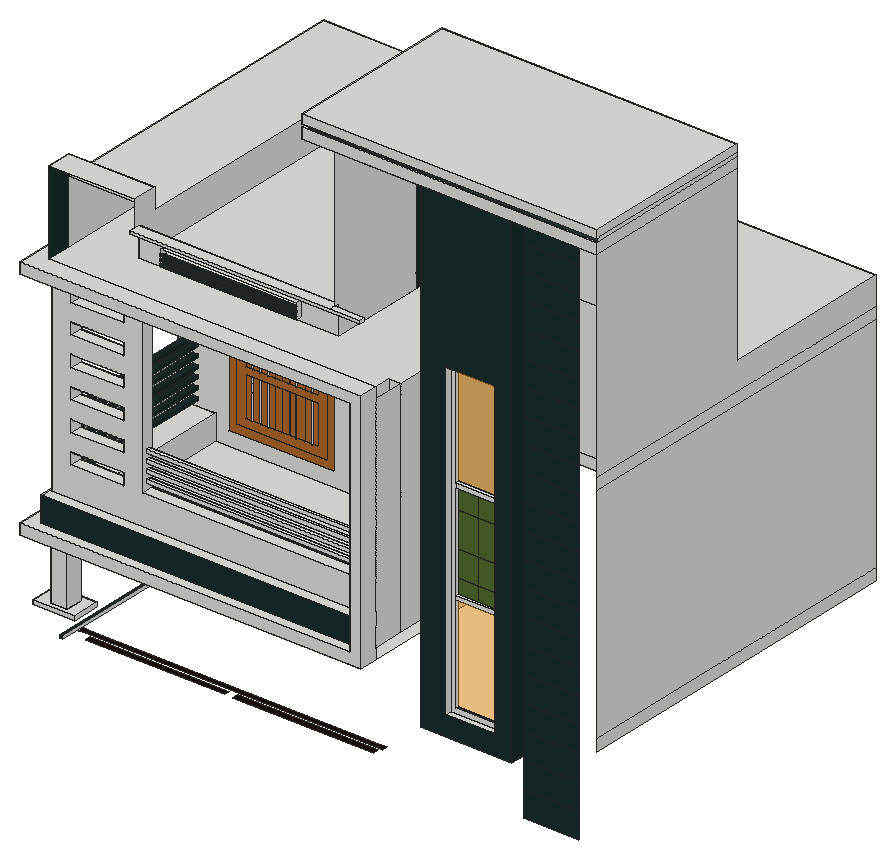
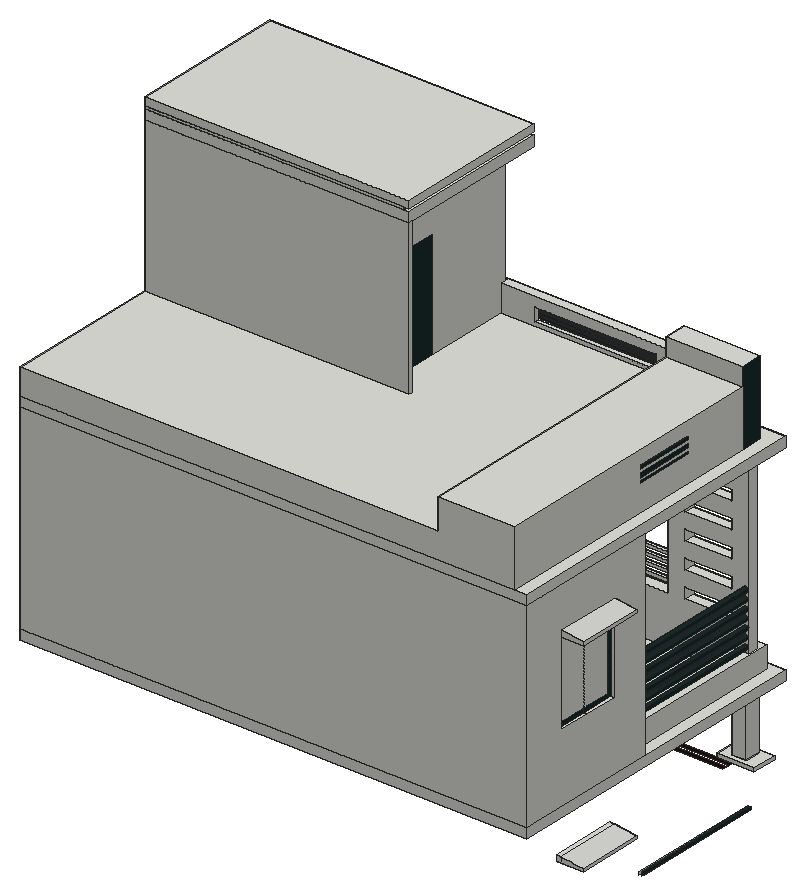
# SketchUp Ruby script. Lengths in inches.
U = 1.inch
M = Sketchup.active_model
def pt(a) = Geom::Point3d.new(a.map { |v| v * U })
def face(e, loops, mat)
  f = e.add_face(loops[0].map { |a| pt(a) })
  loops[1..].each { |l| e.add_face(l.map { |a| pt(a) }).erase! }
  f.material = f.back_material = mat if mat
  f
end
# faces: each face lists its corners as indices into pts; further lists are holes
def faces(e, pts, list, mat = nil) = list.each { |f| face(e, (f[0].is_a?(Array) ? f : [f]).map { |l| l.map { |i| pts[i] } }, mat) }
# xy, xz, yz: faces in a plane at the given z, y or x. An outline is a flat list of corners, or four numbers for a rectangle; further outlines are holes
def ring(l) = l.size == 4 ? [[l[0], l[1]], [l[2], l[1]], [l[2], l[3]], [l[0], l[3]]] : l.each_slice(2).to_a
def flat(e, list, mat, &to3) = list.each { |f| face(e, (f[0].is_a?(Array) ? f : [f]).map { |l| ring(l).map { |u, v| to3.(u, v) } }, mat) }
def xy(e, z, list, mat = nil) = flat(e, list, mat) { |x, y| [x, y, z] }
def xz(e, y, list, mat = nil) = flat(e, list, mat) { |x, z| [x, y, z] }
def yz(e, x, list, mat = nil) = flat(e, list, mat) { |y, z| [x, y, z] }
def lines(e, pts, list) = list.each { |a, b| e.add_line(pt(pts[a]), pt(pts[b])) }
# prism: a flat outline (further loops are holes) pulled along v
def prism(e, loops, v, mat = nil)
  f = face(e, loops, mat); d = Geom::Vector3d.new(v.map { |x| x * U })
  f.pushpull(f.normal.samedirection?(d) ? d.length : -d.length)
end
def box(e, o, s, mat = nil) = prism(e, [[o, [o[0] + s[0], o[1], o[2]], [o[0] + s[0], o[1] + s[1], o[2]], [o[0], o[1] + s[1], o[2]]]], [0, 0, s[2]], mat)
def at(x, y, z, deg = 0) = Geom::Transformation.translation(pt([x, y, z])) * Geom::Transformation.rotation(ORIGIN, Z_AXIS, deg.degrees)
def axes(o, x, y, z) = Geom::Transformation.new([*x, 0, *y, 0, *z, 0, *pt(o).to_a, 1])
def part(name) = M.definitions.add(name)
# library, detail: a bought-in or finely detailed component or shape, given as its bounding box
def library(name, o, s) = part(name).tap { |d| box(d.entities, o, s) }
def detail(e, o, s) = box(e.add_group.entities, o, s)
def put(e, d, t, mat = nil) = e.add_instance(d, t).tap { |i| i.material = mat if mat }
def group(e, t, mat = nil) = e.add_group.tap { |g| g.transformation = t; g.material = mat if mat }.entities
root = M.entities
M.materials.add("[0056_Yellow]").color = [255, 255, 0]
M.materials.add("[0059_DarkOliveGreen]").color = [85, 107, 47]
M.materials.add("[0078_DarkSlateGray]").color = [27, 45, 45]
M.materials.add("[0078_DarkSlateGray]1").color = [47, 79, 79]
M.materials.add("[Translucent Glass Gray]").color = [255, 153, 0]
M.materials["[Translucent Glass Gray]"].alpha = 0.5
M.materials.add("[Wood Bamboo]").color = [177, 105, 43]
M.materials.add("[Wood Veneer 01]").color = [28, 16, 8]
xy(root,66.44,[[15.47,103.41,17.09,183.375]])
xy(root,68.06,[[15.47,103.41,17.09,185.5625]],"[0078_DarkSlateGray]")
xy(root,77.61,[[37.47,93.625,112.35,96.69],[116.92,93.625,192.625,96.69]],"[Wood Veneer 01]")
xy(root,80.73,[[33.97,93.625,37.47,96.69],[37.47,93.625,192.625,96.69],[192.625,93.625,197.375,96.69]],"[Wood Veneer 01]")
xy(root,88.125,[[[12.6875,88.97,35.16,104.16],[13.625,89.97,33.97,103.41]],[[13.625,89.97,33.97,103.41],[20.16,91.68,28.91,100.87]]])
xy(root,90.25,[[[12.6875,88.97,35.16,104.16],[20.16,91.68,28.91,100.87]]])
xy(root,101.9,[[0,208.27,15.875,248.45]])
xy(root,104.5,[[224.51,85.75,273.68,88.9375]])
xy(root,105.36,[[13.625,208.27,16.1875,248.45]])
xy(root,115.35,[[237.85,85.75,264.35,89.1875]])
xy(root,117.75,[[240.25,89.1875,261.95,90.875]])
xy(root,126,[[[13.625,79.375,197.375,185.5625],[97.04,120.8,98.68,120.93,100.24,121.48,101.59,122.42,102.67,123.67,103.375,125.16,103.67,126.78,103.55,128.42,103,129.97,102.0625,131.33,100.81,132.4,99.32,133.11,97.7,133.41,96.06,133.28,94.51,132.73,93.15,131.8,92.08,130.55,91.37,129.06,91.07,127.4375,91.2,125.8,91.75,124.24,92.68,122.88,93.93,121.8125,95.42,121.1],[20.16,91.68,28.91,100.87]]])
xy(root,127,[[97.04,120.8,95.42,121.1,93.93,121.8125,92.68,122.88,91.75,124.24,91.2,125.8,91.07,127.4375,91.37,129.06,92.08,130.55,93.15,131.8,94.51,132.73,96.06,133.28,97.7,133.41,99.32,133.11,100.81,132.4,102.0625,131.33,103,129.97,103.55,128.42,103.67,126.78,103.375,125.16,102.67,123.67,101.59,122.42,100.24,121.48,98.68,120.93]],"[0056_Yellow]")
xy(root,132,[[13.625,79.375,13.625,185.5625,20.7,185.5625,20.7,84.55,191.08,84.55,191.08,79.375],[20.7,84.55,20.7,185.5625,34.04,185.5625,34.04,97,191.08,97,191.08,84.55],[34.04,97,34.04,185.5625,197.375,185.5625,197.375,106,191.08,106,191.08,97]])
xy(root,145.4375,[[20.7,84.55,191.08,84.55,191.08,90.5,21.8,90.5,21.8,97,34.04,97,34.04,185.5625,20.7,185.5625]])
xy(root,148.16,[[21.8,97,24.3,185.5625]])
xy(root,150.1,[[21.8,97,24.3,185.5625]],"[0078_DarkSlateGray]")
xy(root,153.32,[[21.8,97,24.3,185.5625]])
xy(root,155.25,[[21.8,97,24.3,185.5625]],"[0078_DarkSlateGray]")
xy(root,158.47,[[21.8,97,24.3,185.5625]])
xy(root,160.41,[[21.8,97,24.3,185.5625]],"[0078_DarkSlateGray]")
xy(root,161.4375,[[32.21,90.5,60.34,97],[70.54,90.5,191.08,97]])
xy(root,163.63,[[21.8,97,24.3,185.5625]])
xy(root,165.36,[[70.54,92.75,191.08,94.68]])
xy(root,165.57,[[21.8,97,24.3,185.5625]],"[0078_DarkSlateGray]")
xy(root,167.3,[[70.54,92.75,191.08,94.68]])
xy(root,168.0625,[[32.21,90.5,60.34,97]])
xy(root,168.78,[[21.8,97,24.3,185.5625]])
xy(root,169.86,[[240.25,89.1875,261.95,90.875]])
xy(root,170.24,[[70.54,92.75,191.08,94.68]])
xy(root,170.72,[[21.8,97,24.3,185.5625]],"[0078_DarkSlateGray]")
xy(root,172.15,[[240.25,89.1875,261.95,90.875]])
xy(root,172.18,[[70.54,92.75,191.08,94.68]])
xy(root,173.52,[[13.625,208.27,15.875,228.36],[13.625,228.36,15.875,248.45]])
xy(root,173.94,[[21.8,97,24.3,185.5625]])
xy(root,175.11,[[70.54,92.75,191.08,94.68]])
xy(root,175.88,[[21.8,97,24.3,185.5625]],"[0078_DarkSlateGray]")
xy(root,177.05,[[70.54,92.75,191.08,94.68]])
xy(root,177.13,[[32.21,90.5,60.34,97]])
xy(root,179.1,[[21.8,97,24.3,185.5625]])
xy(root,179.99,[[70.54,92.75,191.08,94.68]])
xy(root,181.03,[[21.8,97,24.3,185.5625]],"[0078_DarkSlateGray]")
xy(root,181.93,[[70.54,92.75,191.08,94.68]])
xy(root,183.75,[[32.21,90.5,60.34,97]])
xy(root,192.82,[[32.21,90.5,60.34,97]])
xy(root,199.44,[[32.21,90.5,60.34,97]])
xy(root,208.51,[[32.21,90.5,60.34,97]])
xy(root,215.13,[[32.21,90.5,60.34,97]])
xy(root,224.08,[[240.25,89.1875,261.95,90.875],[0,208.27,15.875,248.45]])
xy(root,224.2,[[32.21,90.5,60.34,97]])
xy(root,226.55,[[240.25,89.1875,261.95,90.875]])
xy(root,230.82,[[32.21,90.5,60.34,97]])
xy(root,239.89,[[32.21,90.5,60.34,97]])
xy(root,246.51,[[32.21,90.5,60.34,97]])
xy(root,252,[[[13.625,79.375,13.625,185.5625,197.375,185.5625,197.375,106,191.08,106,191.08,79.375],[21.8,90.5,70.54,97]]])
xy(root,258,[[13.625,79.375,13.625,274.0625,21.25,274.0625,21.25,88.9375,197.375,88.9375,197.375,79.375]])
xy(root,273.375,[[67.43,91.72,175.33,91.72,175.33,177.76,160.27,177.76,160.27,180.0625,319.25,180.0625,319.25,274.0625,67.43,274.0625]])
xy(root,274.4,[[20.5625,144.23,21.25,180.04]],"[0078_DarkSlateGray]")
xy(root,275.45,[[81.97,88.9375,155.1,91.72]])
xy(root,275.65,[[20.5625,144.23,21.25,180.04]],"[0078_DarkSlateGray]")
xy(root,276.51,[[81.97,87.625,155.1,89.24]])
xy(root,277.51,[[81.97,87.625,155.1,89.24]],"[0078_DarkSlateGray]")
xy(root,277.59,[[20.5625,144.23,21.25,180.04]],"[0078_DarkSlateGray]")
xy(root,278.82,[[81.97,87.625,155.1,89.24]])
xy(root,279.82,[[81.97,87.625,155.1,89.24]],"[0078_DarkSlateGray]")
xy(root,279.95,[[20.5625,144.23,21.25,180.04]],"[0078_DarkSlateGray]")
xy(root,280.95,[[240.25,89.1875,261.95,90.875]])
xy(root,281.2,[[81.97,87.625,155.1,89.24]])
xy(root,282.2,[[81.97,87.625,155.1,89.24]],"[0078_DarkSlateGray]")
xy(root,282.36,[[20.5625,144.23,21.25,180.04]],"[0078_DarkSlateGray]")
xy(root,283.35,[[237.85,85.75,264.35,89.1875]])
xy(root,283.82,[[81.97,88.9375,155.1,91.72]])
xy(root,283.98,[[20.5625,144.23,21.25,180.04]],"[0078_DarkSlateGray]")
xy(root,287.4375,[[67.43,85.75,191.33,88.9375]])
xy(root,289.25,[[67.43,85.75,175.33,91.72],[175.33,85.75,191.33,88.9375]])
xy(root,291.875,[[21.25,102.4,67.43,274.0625]])
xy(root,302.875,[[21.25,88.9375,67.43,102.4]])
xy(root,365.8125,[[160.27,85.75,175.33,177.76],[224.51,85.75,224.51,88.9375,175.33,88.9375,175.33,177.76,160.27,177.76,160.27,180.0625,319.25,180.0625,319.25,85.75,303.01,85.75,303.01,93.625,273.68,93.625,273.68,85.75],[175.33,85.75,224.51,88.9375],[273.68,85.75,303.01,93.625]])
xy(root,371.875,[[160.27,85.75,175.33,85.75,175.33,86.6875,163.33,86.6875,163.33,180.0625,160.27,180.0625],[175.33,85.75,224.51,86.6875],[224.51,85.75,273.68,86.6875],[273.68,85.75,303.01,86.6875],[303.01,85.75,319.25,86.6875],
  [163.33,86.6875,319.25,180.0625]])
xy(root,373.5,[[160.27,85.75,160.27,180.0625,163.33,180.0625,163.33,86.6875,175.33,86.6875,175.33,85.75],[175.33,85.75,224.51,86.6875],[224.51,85.75,273.68,86.6875],[273.68,85.75,303.01,86.6875],[303.01,85.75,319.25,86.6875],
  [163.33,86.6875,319.25,180.0625]])
xy(root,378,[[160.27,85.75,319.25,180.0625]])
xz(root,79.375,[[13.625,126,197.375,126,197.375,258,13.625,258,13.625,252,191.08,252,191.08,132,13.625,132]])
xz(root,84.55,[[20.7,132,191.08,145.4375]],"[0078_DarkSlateGray]")
xz(root,85.75,[[67.43,287.4375,191.33,289.25],[160.27,365.8125,319.25,371.875],[160.27,373.5,319.25,378]])
xz(root,85.75,[[[224.51,104.5,273.68,365.8125],[237.85,115.35,264.35,283.35]]],"[0078_DarkSlateGray]")
xz(root,86.6875,[[163.33,371.875,319.25,373.5]],"[0078_DarkSlateGray]1")
xz(root,87.625,[[81.97,276.51,155.1,277.51],[81.97,278.82,155.1,279.82],[81.97,281.2,155.1,282.2]],"[0078_DarkSlateGray]")
xz(root,88.97,[[12.6875,88.125,35.16,90.25]])
xz(root,89.1875,[[[237.85,115.35,264.35,283.35],[240.25,117.75,261.95,280.95]],[240.25,169.86,261.95,172.15],[240.25,224.08,261.95,226.55]])
xz(root,89.24,[[81.97,276.51,155.1,277.51],[81.97,278.82,155.1,279.82],[81.97,281.2,155.1,282.2]],"[0078_DarkSlateGray]")
xz(root,90.5,[[[21.8,145.4375,191.08,145.4375,191.08,161.4375,70.54,161.4375,70.54,252,21.8,252],[32.21,239.89,60.34,246.51],[32.21,224.2,60.34,230.82],[32.21,208.51,60.34,215.13],[32.21,192.82,60.34,199.44],[32.21,177.13,60.34,183.75],[32.21,161.4375,60.34,168.0625]]])
xz(root,90.875,[[240.25,172.15,251.1,179.83],[251.1,172.15,261.95,179.83],[240.25,179.83,251.1,193.97],[251.1,179.83,261.95,193.97],[240.25,193.97,251.1,212.75],
  [251.1,193.97,261.95,212.75],[240.25,212.75,251.1,224.08],[251.1,212.75,261.95,224.08]],"[0059_DarkOliveGreen]")
xz(root,90.875,[[240.25,117.75,261.95,169.86],[240.25,226.55,261.95,280.95]],"[Translucent Glass Gray]")
xz(root,91.68,[[20.16,88.125,28.91,90.25],[20.16,90.25,28.91,126]])
xz(root,91.72,[[[67.43,273.375,175.33,289.25],[81.97,275.45,155.1,283.82]]])
xz(root,92.75,[[70.54,165.36,191.08,167.3],[70.54,170.24,191.08,172.18],[70.54,175.11,191.08,177.05],[70.54,179.99,191.08,181.93]])
xz(root,93.625,[[273.68,74.39,303.01,88.27],[273.68,88.27,303.01,102.15],[273.68,102.15,303.01,116.03],[273.68,116.03,303.01,129.9],[273.68,129.9,303.01,143.78],
  [273.68,143.78,303.01,157.66],[273.68,157.66,303.01,171.53],[273.68,171.53,303.01,185.41],[273.68,185.41,303.01,199.29],[273.68,199.29,303.01,213.16],
  [273.68,213.16,303.01,227.04],[273.68,227.04,303.01,240.92],[273.68,240.92,303.01,254.8],[273.68,254.8,303.01,268.67],[273.68,268.67,303.01,282.55],
  [273.68,282.55,303.01,296.43],[273.68,296.43,303.01,310.3],[273.68,310.3,303.01,324.18],[273.68,324.18,303.01,338.06],[273.68,338.06,303.01,351.94],
  [273.68,351.94,303.01,365.8125]],"[0078_DarkSlateGray]")
xz(root,94.68,[[70.54,165.36,191.08,167.3],[70.54,170.24,191.08,172.18],[70.54,175.11,191.08,177.05],[70.54,179.99,191.08,181.93]])
xz(root,97,[[[34.04,132,34.04,145.4375,21.8,145.4375,21.8,148.16,24.3,148.16,24.3,150.1,21.8,150.1,21.8,153.32,24.3,153.32,24.3,155.25,21.8,155.25,21.8,158.47,24.3,158.47,24.3,160.41,21.8,160.41,21.8,163.63,24.3,163.63,24.3,165.57,21.8,165.57,21.8,168.78,24.3,168.78,24.3,170.72,21.8,170.72,21.8,173.94,24.3,173.94,24.3,175.88,21.8,175.88,21.8,179.1,24.3,179.1,24.3,181.03,21.8,181.03,21.8,252,70.54,252,70.54,161.4375,191.08,161.4375,191.08,132],[32.21,239.89,60.34,246.51],[32.21,224.2,60.34,230.82],[32.21,208.51,60.34,215.13],[32.21,192.82,60.34,199.44],[32.21,177.13,60.34,183.75],[32.21,161.4375,60.34,168.0625]],[21.8,148.16,24.3,150.1],[21.8,153.32,24.3,155.25],[21.8,158.47,24.3,160.41],[21.8,163.63,24.3,165.57],
  [21.8,168.78,24.3,170.72],[21.8,173.94,24.3,175.88],[21.8,179.1,24.3,181.03]])
xz(root,100.87,[[20.16,88.125,28.91,90.25],[20.16,90.25,28.91,126]])
xz(root,102.4,[[21.25,291.875,67.43,302.875]])
xz(root,104.16,[[12.6875,88.125,35.16,90.25]])
xz(root,106,[[191.08,132,197.375,252]])
xz(root,144.23,[[20.5625,274.4,21.25,275.65],[20.5625,277.59,21.25,279.95],[20.5625,282.36,21.25,283.98]],"[0078_DarkSlateGray]")
xz(root,177.76,[[160.27,273.375,175.33,365.8125]])
xz(root,180.04,[[20.5625,274.4,21.25,275.65],[20.5625,277.59,21.25,279.95],[20.5625,282.36,21.25,283.98]],"[0078_DarkSlateGray]")
xz(root,180.0625,[[160.27,273.375,319.25,365.8125],[160.27,365.8125,319.25,371.875],[163.33,371.875,319.25,373.5],[160.27,373.5,319.25,378]])
xz(root,185.5625,[[[13.625,132,20.7,132,20.7,145.4375,34.04,145.4375,34.04,132,197.375,132,197.375,252,13.625,252],[40.86,139.52,98.43,228.27],[125.82,164.53,182.38,228.72],[21.8,179.1,24.3,181.03],[21.8,173.94,24.3,175.88],[21.8,168.78,24.3,170.72],[21.8,163.63,24.3,165.57],[21.8,158.47,24.3,160.41],[21.8,153.32,24.3,155.25],[21.8,148.16,24.3,150.1]],[20.7,132,34.04,145.4375],[53.48,148.51,53.98,170.01],[57.7,148.51,58.2,170.01],[62.14,148.51,62.64,170.01],
  [65.83,148.51,66.33,170.01],[69.48,148.51,69.98,170.01],[73.23,148.51,73.73,170.01],[77.42,148.51,77.92,170.01],[81.95,148.51,82.45,170.01],
  [85.98,148.51,86.48,170.01],[127.9375,166.65,142.55,226.59],[147.04,166.89,161.16,226.35],[165.89,166.89,180.01,226.35],[53.48,173.46,53.98,173.46,53.96,215.12,53.96,215.27,53.46,215.12],
  [57.7,173.46,58.2,173.46,58.18,215.05,58.18,216.42,57.68,216.3,57.68,215.12],[62.14,173.46,62.64,173.46,62.62,215.05,62.62,217.25,62.12,217.17,62.12,215.12],[65.83,173.46,66.33,173.46,66.3,215.05,66.3,217.65,65.8,217.6,65.8,215.12],[69.48,173.46,69.98,173.46,69.96,215.05,69.96,217.77,69.86,217.78,69.46,217.76,69.46,215.12],[73.23,173.46,73.73,173.46,73.71,215.05,73.71,217.62,73.2,217.67,73.21,215.12],
  [77.42,173.46,77.92,173.46,77.9,215.05,77.9,217.125,77.4,217.21,77.4,215.12],[81.95,173.46,82.45,173.46,82.43,215.05,82.43,216.22,81.93,216.33,81.93,215.12],[85.98,173.46,86.48,173.46,86.46,215.05,86.26,215.12,85.96,215.21,85.96,215.12],[90.46,175.47,91.96,187.59],[92.99,177.37,93.14,177.39,93.27,177.45,93.39,177.53,93.48,177.65,93.54,177.79,93.55,177.93,93.54,178.08,93.48,178.21,93.39,178.33,93.27,178.42,93.14,178.48,92.99,178.49,92.85,178.48,92.71,178.42,92.59,178.33,92.51,178.21,92.45,178.08,92.43,177.93,92.45,177.79,92.51,177.65,92.59,177.53,92.71,177.45,92.85,177.39]])
xz(root,185.5625,[[[40.86,139.52,98.43,228.27],[45.42,144.07,93.87,223.71]],[[45.42,144.07,93.87,223.71],[50.33,173.46,50.33,213.96,53.46,215.12,53.96,215.27,56.66,216.07,57.68,216.3,58.18,216.42,59.91,216.82,62.12,217.17,62.62,217.25,63.2,217.35,65.8,217.6,66.3,217.65,66.53,217.67,69.46,217.76,69.86,217.78,69.96,217.77,73.2,217.67,73.71,217.62,76.52,217.35,77.4,217.21,77.9,217.125,79.8125,216.82,81.93,216.33,82.43,216.22,83.0625,216.07,85.96,215.21,86.26,215.12,86.46,215.05,89.39,213.96,89.39,173.46],[50.375,148.51,89.4375,170.01],[90.46,175.47,91.96,187.59],[92.99,177.37,92.85,177.39,92.71,177.45,92.59,177.53,92.51,177.65,92.45,177.79,92.43,177.93,92.45,178.08,92.51,178.21,92.59,178.33,92.71,178.42,92.85,178.48,92.99,178.49,93.14,178.48,93.27,178.42,93.39,178.33,93.48,178.21,93.54,178.08,93.55,177.93,93.54,177.79,93.48,177.65,93.39,177.53,93.27,177.45,93.14,177.39]],[50.375,148.51,53.48,170.01],[53.98,148.51,57.7,170.01],[58.2,148.51,62.14,170.01],
  [62.64,148.51,65.83,170.01],[66.33,148.51,69.48,170.01],[69.98,148.51,73.23,170.01],[73.73,148.51,77.42,170.01],[77.92,148.51,81.95,170.01],
  [82.45,148.51,85.98,170.01],[86.48,148.51,89.4375,170.01],[[125.82,164.53,144.67,228.72],[127.9375,166.65,142.55,226.59]],[[144.67,164.53,163.53,228.72],[147.04,166.89,161.16,226.35]],[[163.53,164.53,182.38,228.72],[165.89,166.89,180.01,226.35]],
  [50.33,173.46,53.48,173.46,53.46,215.12,50.33,213.96],[53.98,173.46,57.7,173.46,57.68,215.12,57.68,216.3,56.66,216.07,53.96,215.27,53.96,215.12],[58.2,173.46,62.14,173.46,62.12,215.12,62.12,217.17,59.91,216.82,58.18,216.42,58.18,215.05],[62.64,173.46,65.83,173.46,65.8,215.12,65.8,217.6,63.2,217.35,62.62,217.25,62.62,215.05],[66.33,173.46,69.48,173.46,69.46,215.12,69.46,217.76,66.53,217.67,66.3,217.65,66.3,215.05],
  [69.98,173.46,73.23,173.46,73.21,215.12,73.2,217.67,69.96,217.77,69.96,215.05],[73.73,173.46,77.42,173.46,77.4,215.12,77.4,217.21,76.52,217.35,73.71,217.62,73.71,215.05],[77.92,173.46,81.95,173.46,81.93,215.12,81.93,216.33,79.8125,216.82,77.9,217.125,77.9,215.05],[82.45,173.46,85.98,173.46,85.96,215.12,85.96,215.21,83.0625,216.07,82.43,216.22,82.43,215.05],[86.48,173.46,89.39,173.46,89.39,213.96,86.46,215.05]],"[Wood Bamboo]")
xz(root,208.27,[[0,101.9,13.625,101.9,13.625,105.36,0,103.625],[13.625,101.9,16.1875,105.36],[13.625,173.52,15.875,224.08],[0,224.08,13.625,224.08,13.625,227.54,0,225.8125]])
xz(root,248.45,[[0,101.9,0,103.625,13.625,105.36,13.625,101.9],[13.625,101.9,16.1875,105.36],[13.625,173.52,15.875,224.08],[0,224.08,0,225.8125,13.625,227.54,13.625,224.08]])
xz(root,274.0625,[[13.625,126,319.25,132],[13.625,132,319.25,252],[13.625,252,319.25,258],[21.25,258,21.25,291.875,67.43,291.875,67.43,273.375,319.25,273.375,319.25,258]])
yz(root,0,[[208.27,101.9,248.45,103.625],[208.27,224.08,248.45,225.8125]])
yz(root,12.6875,[[88.97,88.125,104.16,90.25]])
yz(root,13.625,[[79.375,126,274.0625,132],[[185.5625,132,274.0625,252],[208.27,173.52,248.45,227.54]],[79.375,252,274.0625,258]])
yz(root,15.47,[[103.41,66.44,185.5625,68.06]],"[0078_DarkSlateGray]")
yz(root,15.875,[[210.84,176.1,228.36,221.5],[228.36,176.1,245.875,221.5]])
yz(root,15.875,[[208.27,173.52,208.27,224.08,228.36,224.08,228.36,221.5,210.84,221.5,210.84,176.1,228.36,176.1,228.36,173.52],[228.36,173.52,228.36,176.1,245.875,176.1,245.875,221.5,228.36,221.5,228.36,224.08,248.45,224.08,248.45,173.52]],"[0078_DarkSlateGray]")
yz(root,17.09,[[103.41,66.44,185.5625,68.06]])
yz(root,20.16,[[91.68,88.125,100.87,90.25],[91.68,90.25,100.87,126]])
yz(root,20.5625,[[144.23,274.4,180.04,275.65],[144.23,277.59,180.04,279.95],[144.23,282.36,180.04,283.98]],"[0078_DarkSlateGray]")
yz(root,20.7,[[84.55,132,185.5625,145.4375]])
yz(root,21.25,[[[102.4,258,274.0625,291.875],[144.23,277.59,180.04,279.95],[144.23,282.36,180.04,283.98],[144.23,274.4,180.04,275.65]]])
yz(root,21.25,[[88.9375,258,102.4,302.875]],"[0078_DarkSlateGray]")
yz(root,21.8,[[90.5,145.4375,97,252]])
yz(root,21.8,[[97,148.16,185.5625,150.1],[97,153.32,185.5625,155.25],[97,158.47,185.5625,160.41],[97,163.63,185.5625,165.57],[97,168.78,185.5625,170.72],
  [97,173.94,185.5625,175.88],[97,179.1,185.5625,181.03]],"[0078_DarkSlateGray]")
yz(root,24.3,[[97,148.16,185.5625,150.1],[97,153.32,185.5625,155.25],[97,158.47,185.5625,160.41],[97,163.63,185.5625,165.57],[97,168.78,185.5625,170.72],
  [97,173.94,185.5625,175.88],[97,179.1,185.5625,181.03]],"[0078_DarkSlateGray]")
yz(root,28.91,[[91.68,88.125,100.87,90.25],[91.68,90.25,100.87,126]])
yz(root,32.21,[[90.5,161.4375,97,168.0625],[90.5,177.13,97,183.75],[90.5,192.82,97,199.44],[90.5,208.51,97,215.13],[90.5,224.2,97,230.82],
  [90.5,239.89,97,246.51]])
yz(root,34.04,[[97,132,185.5625,145.4375]])
yz(root,35.16,[[88.97,88.125,104.16,90.25]])
yz(root,60.34,[[90.5,161.4375,97,168.0625],[90.5,177.13,97,183.75],[90.5,192.82,97,199.44],[90.5,208.51,97,215.13],[90.5,224.2,97,230.82],
  [90.5,239.89,97,246.51]])
yz(root,67.43,[[91.72,273.375,274.0625,273.375,274.0625,291.875,102.4,291.875,102.4,302.875,88.9375,302.875,88.9375,289.25,91.72,289.25],[85.75,287.4375,88.9375,289.25]])
yz(root,70.54,[[[90.5,161.4375,97,252],[92.75,165.36,94.68,167.3],[92.75,170.24,94.68,172.18],[92.75,175.11,94.68,177.05],[92.75,179.99,94.68,181.93]]])
yz(root,81.97,[[88.9375,275.45,91.72,275.45,91.72,283.82,88.9375,283.82,88.9375,282.2,89.24,282.2,89.24,281.2,88.9375,281.2,88.9375,279.82,89.24,279.82,89.24,278.82,88.9375,278.82,88.9375,277.51,89.24,277.51,89.24,276.51,88.9375,276.51]])
yz(root,81.97,[[87.625,276.51,88.9375,277.51],[87.625,278.82,88.9375,279.82],[87.625,281.2,88.9375,282.2]],"[0078_DarkSlateGray]")
yz(root,155.1,[[88.9375,275.45,88.9375,276.51,89.24,276.51,89.24,277.51,88.9375,277.51,88.9375,278.82,89.24,278.82,89.24,279.82,88.9375,279.82,88.9375,281.2,89.24,281.2,89.24,282.2,88.9375,282.2,88.9375,283.82,91.72,283.82,91.72,275.45]])
yz(root,155.1,[[87.625,276.51,88.9375,277.51],[87.625,278.82,88.9375,279.82],[87.625,281.2,88.9375,282.2]],"[0078_DarkSlateGray]")
yz(root,160.27,[[177.76,273.375,180.0625,365.8125],[85.75,365.8125,180.0625,371.875],[85.75,373.5,180.0625,378]])
yz(root,163.33,[[86.6875,371.875,180.0625,373.5]],"[0078_DarkSlateGray]1")
yz(root,175.33,[[91.72,273.375,91.72,289.25,88.9375,289.25,88.9375,365.8125,177.76,365.8125,177.76,338.3125,143.64,338.3125,143.64,273.375]])
yz(root,175.33,[[143.64,273.375,177.76,338.3125]],"[0078_DarkSlateGray]")
yz(root,191.08,[[[79.375,132,79.375,252,106,252,106,132,97,132,97,161.4375,90.5,161.4375,90.5,145.4375,84.55,145.4375,84.55,132],[92.75,179.99,94.68,181.93],[92.75,175.11,94.68,177.05],[92.75,170.24,94.68,172.18],[92.75,165.36,94.68,167.3]],[84.55,132,84.55,145.4375,90.5,145.4375,90.5,161.4375,97,161.4375,97,132]])
yz(root,191.33,[[85.75,287.4375,88.9375,289.25]])
yz(root,197.375,[[79.375,126,88.9375,258],[88.9375,132,106,252],[106,132,185.5625,252]])
yz(root,224.51,[[85.75,104.5,88.9375,365.8125]])
yz(root,237.85,[[85.75,115.35,89.1875,283.35]])
yz(root,240.25,[[89.1875,117.75,90.875,169.86],[89.1875,172.15,90.875,224.08],[89.1875,226.55,90.875,280.95]])
yz(root,261.95,[[89.1875,117.75,90.875,169.86],[89.1875,172.15,90.875,224.08],[89.1875,226.55,90.875,280.95]])
yz(root,264.35,[[85.75,115.35,89.1875,283.35]])
yz(root,273.68,[[85.75,104.5,93.625,365.8125]],"[0078_DarkSlateGray]")
yz(root,319.25,[[85.75,126,274.0625,132],[85.75,132,274.0625,252],[85.75,252,274.0625,258],[85.75,258,274.0625,258,274.0625,273.375,180.0625,273.375,180.0625,365.8125,85.75,365.8125],[85.75,365.8125,180.0625,371.875],
  [86.6875,371.875,180.0625,373.5],[85.75,373.5,180.0625,378]])
p = [[0,208.27,103.625],[13.625,208.27,105.36],[13.625,248.45,105.36],[0,248.45,103.625],[97.04,120.8,126],[95.42,121.1,126],
  [95.42,121.1,127],[97.04,120.8,127],[98.68,120.93,126],[98.68,120.93,127],[100.24,121.48,126],[100.24,121.48,127],
  [93.93,121.8125,126],[93.93,121.8125,127],[101.59,122.42,126],[101.59,122.42,127],[92.68,122.88,126],[92.68,122.88,127],
  [102.67,123.67,126],[102.67,123.67,127],[91.75,124.24,126],[91.75,124.24,127],[103.375,125.16,126],[103.375,125.16,127],
  [91.2,125.8,126],[91.2,125.8,127],[103.67,126.78,126],[103.67,126.78,127],[91.07,127.4375,126],[91.07,127.4375,127],
  [103.55,128.42,126],[103.55,128.42,127],[91.37,129.06,126],[91.37,129.06,127],[103,129.97,126],[103,129.97,127],
  [92.08,130.55,126],[92.08,130.55,127],[102.0625,131.33,126],[102.0625,131.33,127],[93.15,131.8,126],[93.15,131.8,127],
  [100.81,132.4,126],[100.81,132.4,127],[94.51,132.73,126],[94.51,132.73,127],[99.32,133.11,126],[99.32,133.11,127],
  [96.06,133.28,126],[96.06,133.28,127],[97.7,133.41,126],[97.7,133.41,127],[0,208.27,225.8125],[13.625,208.27,227.54],
  [13.625,248.45,227.54],[0,248.45,225.8125]]
faces(root,p,[[0,1,2,3],[52,53,54,55]])
faces(root,p,[[4,5,6,7],[8,4,7,9],[10,8,9,11],[5,12,13,6],[14,10,11,15],[12,16,17,13],[18,14,15,19],[16,20,21,17],
  [22,18,19,23],[20,24,25,21],[26,22,23,27],[24,28,29,25],[30,26,27,31],[28,32,33,29],[34,30,31,35],[32,36,37,33],
  [38,34,35,39],[36,40,41,37],[42,38,39,43],[40,44,45,41],[46,42,43,47],[44,48,49,45],[50,46,47,51],[48,50,51,49]],"[0056_Yellow]")
